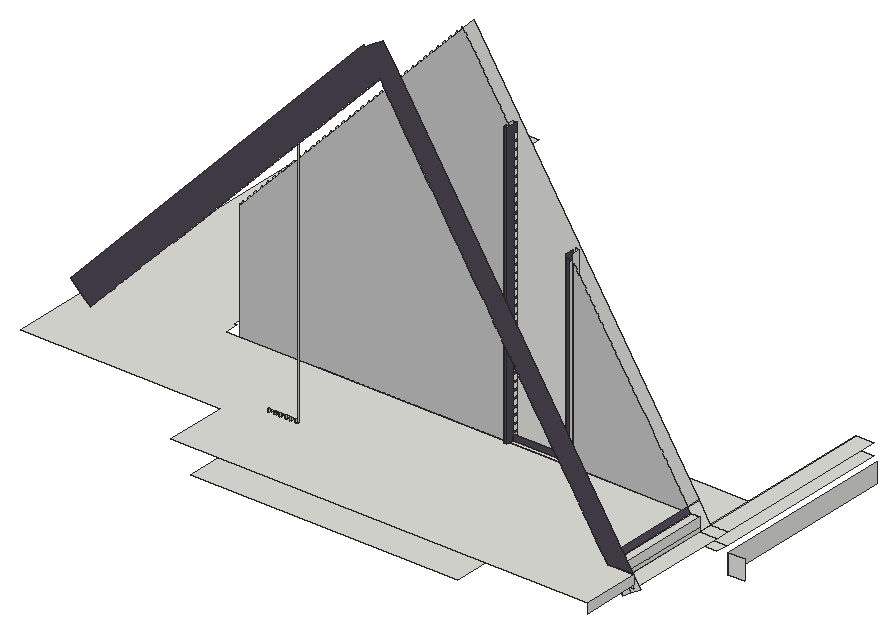
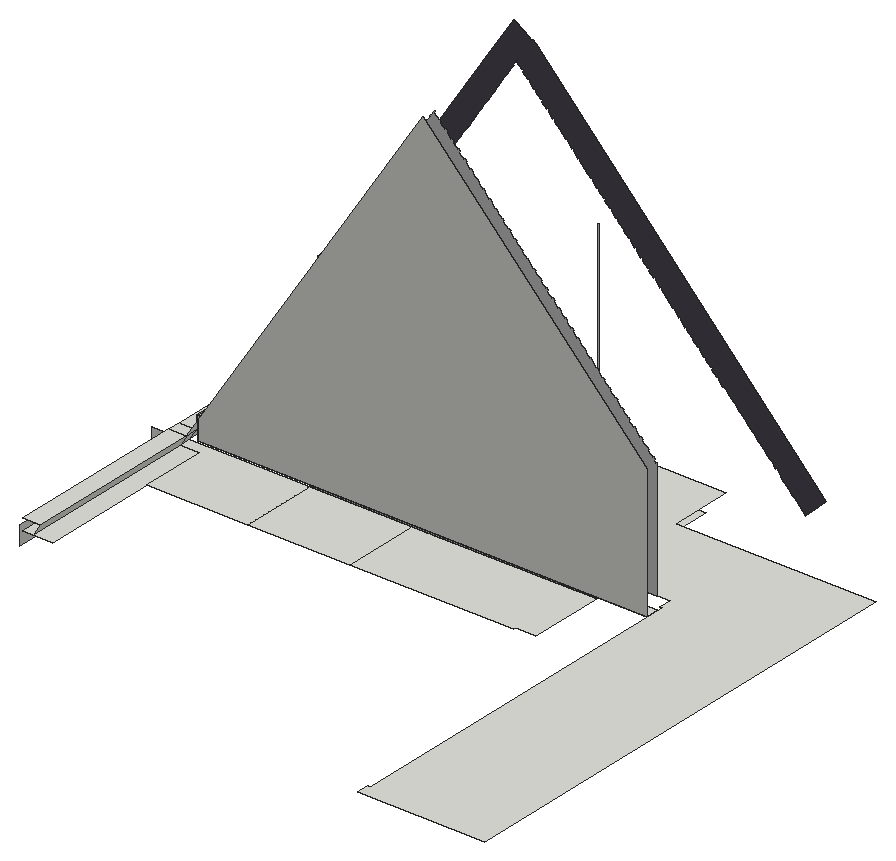
# SketchUp Ruby script. Lengths in inches.
U = 1.inch
M = Sketchup.active_model
def pt(a) = Geom::Point3d.new(a.map { |v| v * U })
def face(e, loops, mat)
  f = e.add_face(loops[0].map { |a| pt(a) })
  loops[1..].each { |l| e.add_face(l.map { |a| pt(a) }).erase! }
  f.material = f.back_material = mat if mat
  f
end
# faces: each face lists its corners as indices into pts; further lists are holes
def faces(e, pts, list, mat = nil) = list.each { |f| face(e, (f[0].is_a?(Array) ? f : [f]).map { |l| l.map { |i| pts[i] } }, mat) }
# xy, xz, yz: faces in a plane at the given z, y or x. An outline is a flat list of corners, or four numbers for a rectangle; further outlines are holes
def ring(l) = l.size == 4 ? [[l[0], l[1]], [l[2], l[1]], [l[2], l[3]], [l[0], l[3]]] : l.each_slice(2).to_a
def flat(e, list, mat, &to3) = list.each { |f| face(e, (f[0].is_a?(Array) ? f : [f]).map { |l| ring(l).map { |u, v| to3.(u, v) } }, mat) }
def xy(e, z, list, mat = nil) = flat(e, list, mat) { |x, y| [x, y, z] }
def xz(e, y, list, mat = nil) = flat(e, list, mat) { |x, z| [x, y, z] }
def yz(e, x, list, mat = nil) = flat(e, list, mat) { |y, z| [x, y, z] }
def lines(e, pts, list) = list.each { |a, b| e.add_line(pt(pts[a]), pt(pts[b])) }
# prism: a flat outline (further loops are holes) pulled along v
def prism(e, loops, v, mat = nil)
  f = face(e, loops, mat); d = Geom::Vector3d.new(v.map { |x| x * U })
  f.pushpull(f.normal.samedirection?(d) ? d.length : -d.length)
end
def box(e, o, s, mat = nil) = prism(e, [[o, [o[0] + s[0], o[1], o[2]], [o[0] + s[0], o[1] + s[1], o[2]], [o[0], o[1] + s[1], o[2]]]], [0, 0, s[2]], mat)
def at(x, y, z, deg = 0) = Geom::Transformation.translation(pt([x, y, z])) * Geom::Transformation.rotation(ORIGIN, Z_AXIS, deg.degrees)
def axes(o, x, y, z) = Geom::Transformation.new([*x, 0, *y, 0, *z, 0, *pt(o).to_a, 1])
def part(name) = M.definitions.add(name)
# library, detail: a bought-in or finely detailed component or shape, given as its bounding box
def library(name, o, s) = part(name).tap { |d| box(d.entities, o, s) }
def detail(e, o, s) = box(e.add_group.entities, o, s)
def put(e, d, t, mat = nil) = e.add_instance(d, t).tap { |i| i.material = mat if mat }
def group(e, t, mat = nil) = e.add_group.tap { |g| g.transformation = t; g.material = mat if mat }.entities
root = M.entities
M.materials.add("[Color M02]").color = [198, 198, 198]
M.materials.add("[Color M06]").color = [79, 71, 84]
c1 = library("A$C06767DEF\#1",[-8.3,1.21,0],[7.09,7.09,5.51])
xy(root,250.875,[[[1365.01,437.0625,1365.01,509.6875,1451.49,509.6875,1451.49,521.5625,1504.89,521.5625,1504.89,437.0625],[1470.93,456.39,1472.48,456.6,1473.93,457.2,1475.17,458.15,1476.12,459.39,1476.72,460.84,1476.93,462.39,1476.72,463.95,1476.12,465.39,1475.17,466.64,1473.93,467.59,1472.48,468.1875,1470.93,468.39,1469.375,468.1875,1467.93,467.59,1466.68,466.64,1465.73,465.39,1465.13,463.95,1464.93,462.39,1465.13,460.84,1465.73,459.39,1466.68,458.15,1467.93,457.2,1469.375,456.6],[1407.85,459.39,1409.4,459.6,1410.85,460.2,1412.09,461.15,1413.04,462.39,1413.64,463.84,1413.85,465.39,1413.64,466.95,1413.04,468.39,1412.09,469.64,1410.85,470.59,1409.4,471.1875,1407.85,471.39,1406.3,471.1875,1404.85,470.59,1403.61,469.64,1402.65,468.39,1402.05,466.95,1401.85,465.39,1402.05,463.84,1402.65,462.39,1403.61,461.15,1404.85,460.2,1406.3,459.6]]])
xy(root,251.0625,[[1365.01,509.6875,1451.49,521.5625],[1354.48,521.5625,1354.48,561.375,1365.24,561.375,1365.24,562.32,1451.49,562.32,1451.49,521.5625],[1451.49,521.5625,1504.89,562.32],[1504.89,521.5625,1504.89,562.32,1557.79,562.32,1557.79,527.76,1573.31,527.76,1573.31,521.5625],[1557.79,527.76,1573.31,623.84]])
xy(root,252.25,[[1470.93,456.39,1469.375,456.6,1467.93,457.2,1466.68,458.15,1465.73,459.39,1465.13,460.84,1464.93,462.39,1465.13,463.95,1465.73,465.39,1466.68,466.64,1467.93,467.59,1469.375,468.1875,1470.93,468.39,1472.48,468.1875,1473.93,467.59,1475.17,466.64,1476.12,465.39,1476.72,463.95,1476.93,462.39,1476.72,460.84,1476.12,459.39,1475.17,458.15,1473.93,457.2,1472.48,456.6]])
xy(root,252.375,[[1407.85,459.39,1406.3,459.6,1404.85,460.2,1403.61,461.15,1402.65,462.39,1402.05,463.84,1401.85,465.39,1402.05,466.95,1402.65,468.39,1403.61,469.64,1404.85,470.59,1406.3,471.1875,1407.85,471.39,1409.4,471.1875,1410.85,470.59,1412.09,469.64,1413.04,468.39,1413.64,466.95,1413.85,465.39,1413.64,463.84,1413.04,462.39,1412.09,461.15,1410.85,460.2,1409.4,459.6]])
xy(root,257.0625,[[1563.99,467.1875,1573.31,521.5625],[1322.96,521.5625,1557.92,528.48],[1563.99,521.5625,1573.31,528.48],[1563.99,528.48,1573.31,623.84]])
xy(root,259.68,[[1371.61,480.14,1373.93,480.77],[1374.53,480.14,1376.84,480.77],[1377.4375,480.14,1379.75,480.77],[1380.35,480.14,1382.66,480.77],[1383.26,480.14,1385.58,480.77]])
xy(root,262,[[1371.61,480.14,1373.93,480.77],[1374.53,480.14,1376.84,480.77],[1377.4375,480.14,1379.75,480.77],[1380.35,480.14,1382.66,480.77],[1383.26,480.14,1385.58,480.77]])
xy(root,262.73,[[1371.64,480.14,1373.96,480.77],[1374.56,480.14,1376.87,480.77],[1377.47,480.14,1379.78,480.77],[1380.38,480.14,1382.69,480.77],[1383.29,480.14,1385.6,480.77]])
xy(root,263.89,[[[1354.48,437.0625,1573.31,437.0625,1573.31,467.1875,1563.99,467.1875,1563.99,521.5625,1497.36,521.5625,1497.36,519.6875,1495.49,519.6875,1495.49,521.5625,1464.52,521.5625,1464.52,519.6875,1462.77,519.6875,1462.77,521.5625,1316.04,521.5625,1316.04,528.48,1314.46,528.48,1314.46,719.59,1316.04,719.59,1316.04,726.125,1249.48,726.125,1249.48,469.875,1354.48,469.875],[1317.4375,480.14,1386.75,480.77]],[1462.77,519.6875,1464.52,521.5625],[1495.49,519.6875,1497.36,521.5625],[1462.77,521.5625,1464.52,526.125],[1464.52,521.5625,1495.49,523.75],
  [1495.49,521.5625,1497.36,526.125]])
xy(root,265.04,[[1371.64,480.14,1373.96,480.77],[1374.56,480.14,1376.87,480.77],[1377.47,480.14,1379.78,480.77],[1380.38,480.14,1382.69,480.77],[1383.29,480.14,1385.6,480.77]])
xz(root,467.1875,[[1567.23,252.01,1571.28,254.61,1569.71,257.0625,1563.99,257.0625],[1571.28,254.61,1576.55,257.98,1573.31,263.03,1573.31,257.0625,1569.71,257.0625],[1563.99,257.0625,1569.71,258.95],[1569.71,257.0625,1573.31,258.95],[1563.99,258.95,1569.71,263.89],
  [1569.71,258.95,1573.31,258.95,1573.31,263.03,1572.76,263.89,1569.71,263.89],[1573.31,263.03,1572.76,263.89,1573.31,263.89]])
xz(root,467.1875,[[1563.99,257.0625,1563.99,263.89,1572.76,263.89,1449.33,456.41,1441.66,468.38,1436.39,465.01,1432,462.19,1431.44,462.72,1430.11,461.31,1277.91,299.61,1285.45,292.52,1288.59,289.56,1291.01,292.13,1291.88,293.0625,1294.3,295.64,1295.18,296.57,1297.6,299.14,1298.48,300.07,1300.9,302.64,1301.78,303.58,1301.55,303.79,1303.97,306.36,1304.2,306.15,1305.08,307.08,1304.85,307.29,1307.27,309.87,1307.5,309.65,1308.375,310.59,1310.8,313.16,1311.68,314.09,1314.1,316.66,1314.97,317.59,1317.39,320.17,1318.27,321.1,1320.69,323.67,1321.57,324.6,1323.99,327.17,1324.87,328.11,1327.29,330.68,1328.17,331.61,1330.59,334.18,1331.47,335.11,1331.92,334.6875,1334.34,337.26,1333.89,337.6875,1334.76,338.62,1335.22,338.19,1337.64,340.76,1337.1875,341.19,1338.0625,342.125,1338.52,341.69,1340.94,344.27,1340.48,344.7,1341.36,345.63,1341.82,345.2,1344.24,347.77,1343.78,348.2,1344.66,349.13,1345.12,348.7,1347.54,351.28,1347.08,351.7,1347.96,352.64,1348.41,352.21,1350.84,354.78,1350.38,355.21,1351.26,356.14,1351.71,355.71,1354.13,358.28,1353.68,358.71,1354.56,359.64,1355.01,359.22,1357.43,361.79,1356.98,362.22,1357.85,363.15,1358.31,362.72,1360.73,365.29,1360.28,365.72,1361.15,366.65,1361.61,366.22,1364.03,368.8,1363.57,369.23,1364.45,370.16,1364.91,369.73,1367.33,372.3,1366.87,372.73,1367.75,373.66,1368.21,373.23,1370.625,375.81,1370.17,376.23,1371.05,377.17,1371.5,376.74,1373.92,379.31,1373.47,379.74,1374.35,380.67,1374.8,380.24,1377.22,382.8125,1376.77,383.24,1377.65,384.17,1378.1,383.75,1380.52,386.32,1380.07,386.75,1380.94,387.68,1381.4,387.25,1383.82,389.82,1383.37,390.25,1384.24,391.18,1384.7,390.75,1387.12,393.33,1386.66,393.75,1387.54,394.6875,1388,394.26,1390.42,396.83,1389.96,397.26,1390.84,398.19,1391.3,397.76,1393.72,400.34,1393.26,400.76,1394.14,401.7,1394.59,401.27,1397.01,403.84,1396.56,404.27,1397.4375,405.2,1397.89,404.77,1400.3125,407.34,1399.86,407.77,1400.74,408.7,1401.19,408.28,1403.61,410.85,1403.16,411.28,1404.03,412.21,1404.49,411.78,1406.91,414.35,1406.46,414.78,1407.33,415.71,1407.79,415.28,1410.21,417.86,1409.75,418.28,1410.63,419.22,1411.09,418.79,1413.51,421.36,1413.05,421.79,1413.93,422.72,1414.38,422.29,1416.81,424.86,1416.35,425.29,1417.23,426.23,1417.68,425.8,1420.1,428.37,1419.65,428.8,1420.53,429.73,1420.98,429.3,1423.4,431.875,1422.95,432.3,1423.83,433.23,1424.28,432.81,1426.7,435.38,1426.25,435.81,1427.125,436.74,1427.58,436.31,1430,438.88,1429.55,439.31,1430.42,440.24,1430.88,439.8125,1433.3,442.39,1432.84,442.8125,1433.72,443.75,1434.18,443.32,1436.6,445.89,1436.14,446.32,1437.02,447.25,1437.47,446.82,1439.9,449.39,1439.44,449.82,1439.71,450.11,1440.02,450.4375,1441.59,447.99,1442.09,447.21,1441.72,446.98,1443.41,444.33,1443.78,444.57,1444.28,443.79,1443.91,443.56,1445.61,440.91,1445.97,441.15,1446.47,440.375,1446.1,440.14,1447.8,437.49,1448.17,437.73,1448.66,436.95,1448.3,436.72,1449.99,434.07,1450.36,434.31,1450.86,433.53,1450.49,433.3,1452.18,430.65,1452.55,430.89,1453.05,430.11,1452.68,429.88,1454.375,427.23,1454.74,427.47,1455.24,426.69,1454.875,426.46,1456.57,423.8125,1456.9375,424.05,1457.43,423.27,1457.07,423.04,1458.76,420.39,1459.13,420.63,1459.63,419.85,1459.26,419.62,1460.95,416.97,1461.32,417.21,1461.82,416.43,1461.45,416.2,1463.15,413.55,1463.51,413.79,1464.01,413.01,1463.64,412.78,1465.34,410.13,1465.71,410.37,1466.2,409.59,1465.84,409.36,1467.53,406.71,1467.9,406.95,1468.4,406.17,1468.03,405.9375,1469.72,403.29,1470.09,403.53,1470.59,402.75,1470.22,402.52,1471.92,399.875,1472.28,400.11,1472.78,399.33,1472.41,399.1,1474.11,396.45,1474.48,396.69,1474.98,395.91,1474.61,395.68,1476.3,393.03,1476.67,393.27,1477.17,392.49,1476.8,392.26,1478.49,389.61,1478.86,389.85,1479.36,389.07,1478.99,388.84,1480.6875,386.19,1481.05,386.43,1481.55,385.65,1481.18,385.42,1482.88,382.77,1483.25,383.01,1483.75,382.23,1483.38,382,1485.07,379.35,1485.44,379.59,1485.9375,378.8125,1485.57,378.58,1487.26,375.93,1487.63,376.17,1488.13,375.39,1487.76,375.16,1489.46,372.51,1489.83,372.75,1490.32,371.97,1489.96,371.74,1491.65,369.09,1492.02,369.33,1492.65,368.34,1492.28,368.11,1493.98,365.46,1494.35,365.7,1494.98,364.71,1496.67,362.07,1497.31,361.08,1496.9375,360.85,1498.63,358.2,1499,358.4375,1499.63,357.45,1499.27,357.22,1500.96,354.57,1501.33,354.81,1501.96,353.82,1501.59,353.58,1503.29,350.94,1503.66,351.18,1504.29,350.19,1503.92,349.95,1505.61,347.3125,1505.98,347.55,1506.62,346.56,1506.25,346.32,1507.94,343.68,1508.3125,343.92,1508.94,342.93,1508.58,342.69,1510.27,340.05,1510.64,340.29,1511.17,339.46,1510.8,339.22,1512.5,336.58,1512.86,336.8125,1513.4,335.98,1513.03,335.75,1514.72,333.11,1515.09,333.34,1515.62,332.51,1515.25,332.28,1516.95,329.63,1517.32,329.87,1517.85,329.04,1517.48,328.8,1519.18,326.16,1519.54,326.4,1520.08,325.57,1519.71,325.33,1521.4,322.6875,1521.77,322.92,1522.3,322.09,1521.93,321.86,1523.63,319.21,1524,319.45,1524.53,318.62,1524.16,318.38,1525.85,315.74,1526.22,315.98,1526.75,315.15,1526.39,314.91,1528.08,312.27,1528.45,312.51,1528.98,311.68,1528.61,311.44,1530.31,308.8,1530.68,309.03,1531.21,308.2,1530.84,307.97,1532.53,305.32,1532.9,305.56,1533.43,304.73,1533.07,304.49,1534.76,301.85,1535.13,302.09,1535.66,301.26,1535.4,301.09,1537.09,298.45,1537.35,298.61,1537.89,297.79,1537.62,297.62,1539.32,294.97,1539.58,295.14,1540.11,294.3125,1539.85,294.14,1541.54,291.5,1541.81,291.67,1542.34,290.84,1542.08,290.67,1543.77,288.03,1544.03,288.2,1544.56,287.37,1544.3,287.2,1546,284.56,1546.26,284.72,1546.79,283.89,1546.53,283.73,1548.22,281.08,1548.49,281.25,1549.02,280.42,1548.75,280.25,1550.45,277.61,1550.71,277.78,1551.24,276.95,1550.98,276.78,1552.68,274.14,1552.9375,274.31,1553.47,273.48,1553.21,273.31,1554.9,270.67,1555.16,270.83,1555.7,270,1555.43,269.84,1557.13,267.19,1557.39,267.36,1557.92,266.53,1557.66,266.36,1559.35,263.72,1559.62,263.89]],"[Color M06]")
xz(root,480.14,[[1386.17,258.95,1386.75,263.89],[1371.64,262.73,1373.96,263.89],[1374.56,262.73,1376.87,263.89],[1377.47,262.73,1379.78,263.89],[1380.38,262.73,1382.69,263.89],
  [1383.29,262.73,1385.6,263.89]])
xz(root,480.77,[[1371.64,262.73,1373.96,263.89],[1374.56,262.73,1376.87,263.89],[1377.47,262.73,1379.78,263.89],[1380.38,262.73,1382.69,263.89],[1383.29,262.73,1385.6,263.89]])
xz(root,509.6875,[[1365.01,250.875,1451.49,251.0625]])
xz(root,519.6875,[[1462.77,263.89,1464.52,412.22],[1495.49,263.89,1497.36,263.89,1497.36,360.99,1496.99,360.76,1496.9375,360.85,1497.31,361.08,1496.67,362.07,1496.3,361.83,1495.49,363.11]],"[Color M06]")
xz(root,521.5625,[[1451.49,250.875,1504.89,251.0625],[1365.01,251.0625,1504.89,257.0625],[1365.01,257.0625,1504.89,258.95],[1504.89,257.0625,1557.92,258.95],[1557.92,257.0625,1563.99,257.0625,1562.78,258.95,1557.92,258.95],
  [1563.99,257.0625,1562.78,258.95,1563.99,258.95],[1365.01,258.95,1504.89,263.89],[1504.89,258.95,1557.92,263.89],[1557.92,258.95,1562.78,258.95,1559.62,263.89,1559.35,263.72,1559.25,263.89,1557.92,263.89],[1562.78,258.95,1559.62,263.89,1562.78,263.89],
  [1562.78,258.95,1563.99,263.89],[1559.35,263.72,1559.25,263.89,1559.62,263.89],[1557.92,263.89,1559.25,263.89,1557.92,265.95],[1559.25,263.89,1559.62,263.89,1557.92,266.53,1557.92,265.95]])
xz(root,521.5625,[[1322.96,263.89,1462.77,263.89,1462.77,412.22,1464,412.22,1463.7,412.6875,1464.07,412.92,1463.51,413.79,1463.15,413.55,1461.96,415.41,1461.51,416.11,1461.875,416.34,1461.32,417.21,1460.95,416.97,1459.77,418.83,1459.32,419.53,1459.68,419.76,1459.13,420.63,1458.76,420.39,1457.57,422.25,1457.12,422.95,1457.49,423.18,1456.9375,424.05,1456.57,423.8125,1455.38,425.67,1454.93,426.37,1455.3,426.6,1454.74,427.47,1454.375,427.23,1453.1875,429.09,1452.74,429.79,1453.11,430.02,1452.55,430.89,1452.18,430.65,1451,432.51,1450.55,433.21,1450.91,433.44,1450.36,434.31,1449.99,434.07,1448.8,435.93,1448.35,436.63,1448.72,436.86,1448.17,437.73,1447.8,437.49,1446.61,439.35,1446.16,440.05,1446.53,440.28,1445.97,441.15,1445.61,440.91,1444.42,442.77,1443.97,443.47,1444.34,443.7,1443.78,444.57,1443.41,444.33,1442.22,446.1875,1441.77,446.89,1442.14,447.125,1441.59,447.99,1441.22,447.75,1440.03,449.61,1439.71,450.11,1439.44,449.82,1439.9,449.39,1437.47,446.82,1437.02,447.25,1436.14,446.32,1436.6,445.89,1434.18,443.32,1433.72,443.75,1432.84,442.8125,1433.3,442.39,1430.88,439.8125,1430.42,440.24,1429.55,439.31,1430,438.88,1427.58,436.31,1427.125,436.74,1426.25,435.81,1426.7,435.38,1424.28,432.81,1423.83,433.23,1422.95,432.3,1423.4,431.875,1420.98,429.3,1420.53,429.73,1419.65,428.8,1420.1,428.37,1417.68,425.8,1417.23,426.23,1416.35,425.29,1416.81,424.86,1414.38,422.29,1413.93,422.72,1413.05,421.79,1413.51,421.36,1411.09,418.79,1410.63,419.22,1409.75,418.28,1410.21,417.86,1407.79,415.28,1407.33,415.71,1406.46,414.78,1406.91,414.35,1404.49,411.78,1404.03,412.21,1403.16,411.28,1403.61,410.85,1401.19,408.28,1400.74,408.7,1399.86,407.77,1400.3125,407.34,1397.89,404.77,1397.4375,405.2,1396.56,404.27,1397.01,403.84,1394.59,401.27,1394.14,401.7,1393.26,400.76,1393.72,400.34,1391.3,397.76,1390.84,398.19,1389.96,397.26,1390.42,396.83,1388,394.26,1387.54,394.6875,1386.66,393.75,1387.12,393.33,1384.7,390.75,1384.24,391.18,1383.37,390.25,1383.82,389.82,1381.4,387.25,1380.94,387.68,1380.07,386.75,1380.52,386.32,1378.1,383.75,1377.65,384.17,1376.77,383.24,1377.22,382.8125,1374.8,380.24,1374.35,380.67,1373.47,379.74,1373.92,379.31,1371.5,376.74,1371.05,377.17,1370.17,376.23,1370.625,375.81,1368.21,373.23,1367.75,373.66,1366.87,372.73,1367.33,372.3,1364.91,369.73,1364.45,370.16,1363.57,369.23,1364.03,368.8,1361.61,366.22,1361.15,366.65,1360.28,365.72,1360.73,365.29,1358.31,362.72,1357.85,363.15,1356.98,362.22,1357.43,361.79,1355.01,359.22,1354.56,359.64,1353.68,358.71,1354.13,358.28,1351.71,355.71,1351.26,356.14,1350.38,355.21,1350.84,354.78,1348.41,352.21,1347.96,352.64,1347.08,351.7,1347.54,351.28,1345.12,348.7,1344.66,349.13,1343.78,348.2,1344.24,347.77,1341.82,345.2,1341.36,345.63,1340.48,344.7,1340.94,344.27,1338.52,341.69,1338.0625,342.125,1337.1875,341.19,1337.64,340.76,1337.04,340.125,1336.64,339.7,1335.22,338.19,1334.76,338.62,1333.89,337.6875,1334.34,337.26,1331.92,334.6875,1331.47,335.11,1330.59,334.18,1331.04,333.75,1328.62,331.18,1328.17,331.61,1327.29,330.68,1327.75,330.25,1325.32,327.68,1324.87,328.11,1323.99,327.17,1324.45,326.75,1323.42,325.65,1322.96,326.08],[1497.36,263.89,1557.92,263.89,1557.92,265.95,1557.66,266.36,1557.92,266.53,1557.39,267.36,1557.13,267.19,1555.43,269.84,1555.7,270,1555.16,270.83,1554.9,270.67,1553.21,273.31,1553.47,273.48,1552.9375,274.31,1552.68,274.14,1550.98,276.78,1551.24,276.95,1550.71,277.78,1550.45,277.61,1548.75,280.25,1549.02,280.42,1548.49,281.25,1548.22,281.08,1546.53,283.73,1546.79,283.89,1546.26,284.72,1546,284.56,1544.3,287.2,1544.56,287.37,1544.03,288.2,1543.77,288.03,1542.08,290.67,1542.34,290.84,1541.81,291.67,1541.54,291.5,1539.85,294.14,1540.11,294.3125,1539.58,295.14,1537.89,297.79,1537.35,298.61,1535.66,301.26,1535.13,302.09,1534.76,301.85,1533.07,304.49,1533.43,304.73,1532.9,305.56,1532.53,305.32,1530.84,307.97,1531.21,308.2,1530.68,309.03,1530.31,308.8,1528.61,311.44,1528.98,311.68,1528.45,312.51,1528.08,312.27,1526.39,314.91,1526.75,315.15,1526.22,315.98,1525.85,315.74,1524.16,318.38,1524.53,318.62,1524,319.45,1523.63,319.21,1521.93,321.86,1522.3,322.09,1521.77,322.92,1521.4,322.6875,1519.71,325.33,1520.08,325.57,1519.54,326.4,1519.18,326.16,1517.48,328.8,1517.85,329.04,1517.32,329.87,1516.95,329.63,1515.25,332.28,1515.62,332.51,1515.09,333.34,1514.72,333.11,1513.03,335.75,1513.4,335.98,1512.86,336.8125,1512.5,336.58,1510.8,339.22,1511.17,339.46,1510.74,340.125,1510.64,340.29,1510.27,340.05,1508.58,342.69,1508.94,342.93,1508.3125,343.92,1507.94,343.68,1506.25,346.32,1506.62,346.56,1505.98,347.55,1505.61,347.3125,1503.92,349.95,1504.29,350.19,1503.66,351.18,1503.29,350.94,1501.59,353.58,1501.96,353.82,1501.33,354.81,1500.96,354.57,1499.27,357.22,1499.63,357.45,1499,358.4375,1498.63,358.2,1497.36,360.18]],"[Color M02]")
xz(root,523.31,[[1577.59,240.88,1586.28,251.0625]])
xz(root,523.75,[[1464.52,263.89,1495.49,267.02]],"[Color M06]")
xz(root,526.125,[[1462.77,263.89,1464.52,412.22],[1495.49,263.89,1497.36,363.92]])
xz(root,528.48,[[1322.96,257.0625,1322.96,326.08,1440.02,450.4375,1557.92,266.53,1557.92,257.0625]])
yz(root,1371.04,[[480.14,262.73,480.77,265.04]])
yz(root,1371.61,[[480.14,259.68,480.77,262]])
yz(root,1371.64,[[480.14,262.73,480.77,265.04]])
yz(root,1373.93,[[480.14,259.68,480.77,262]])
yz(root,1373.96,[[480.14,262.73,480.77,265.04]])
yz(root,1374.53,[[480.14,259.68,480.77,262]])
yz(root,1374.56,[[480.14,262.73,480.77,265.04]])
yz(root,1376.84,[[480.14,259.68,480.77,262]])
yz(root,1376.87,[[480.14,262.73,480.77,265.04]])
yz(root,1377.4375,[[480.14,259.68,480.77,262]])
yz(root,1377.47,[[480.14,262.73,480.77,265.04]])
yz(root,1379.75,[[480.14,259.68,480.77,262]])
yz(root,1379.78,[[480.14,262.73,480.77,265.04]])
yz(root,1380.35,[[480.14,259.68,480.77,262]])
yz(root,1380.38,[[480.14,262.73,480.77,265.04]])
yz(root,1382.66,[[480.14,259.68,480.77,262]])
yz(root,1382.69,[[480.14,262.73,480.77,265.04]])
yz(root,1383.26,[[480.14,259.68,480.77,262]])
yz(root,1383.29,[[480.14,262.73,480.77,265.04]])
yz(root,1385.58,[[480.14,259.68,480.77,262]])
yz(root,1385.6,[[480.14,262.73,480.77,265.04]])
yz(root,1386.75,[[480.14,258.95,480.77,263.89],[480.14,263.89,480.77,397.75]])
yz(root,1451.49,[[509.6875,250.875,521.5625,251.0625]])
yz(root,1462.77,[[521.5625,263.89,526.125,412.22]])
yz(root,1462.77,[[519.6875,263.89,521.5625,412.22]],"[Color M06]")
yz(root,1464.52,[[523.75,263.89,526.125,267.02]])
yz(root,1464.52,[[519.6875,263.89,523.75,263.89,523.75,267.02,526.125,267.02,526.125,267.83,523.75,267.83,523.75,270.95,526.125,270.95,526.125,271.76,523.75,271.76,523.75,274.89,526.125,274.89,526.125,275.7,523.75,275.7,523.75,278.83,526.125,278.83,526.125,279.64,523.75,279.64,523.75,282.77,526.125,282.77,526.125,283.58,523.75,283.58,523.75,286.7,526.125,286.7,526.125,287.51,523.75,287.51,523.75,290.64,526.125,290.64,526.125,291.45,523.75,291.45,523.75,294.58,526.125,294.58,526.125,295.39,523.75,295.39,523.75,298.52,526.125,298.52,526.125,299.33,523.75,299.33,523.75,302.45,526.125,302.45,526.125,303.26,523.75,303.26,523.75,306.39,526.125,306.39,526.125,307.2,523.75,307.2,523.75,310.33,526.125,310.33,526.125,311.14,523.75,311.14,523.75,314.27,526.125,314.27,526.125,315.08,524.25,315.08,524.25,318.2,526.125,318.2,526.125,319.01,524.25,319.01,524.25,322.14,526.125,322.14,526.125,322.89,524.25,322.89,524.25,326.02,526.125,326.02,526.125,326.76,524.25,326.76,524.25,329.89,526.125,329.89,526.125,330.64,524.25,330.64,524.25,333.77,526.125,333.77,526.125,334.51,524.25,334.51,524.25,337.64,526.125,337.64,526.125,338.39,524.25,338.39,524.25,341.52,526.125,341.52,526.125,341.93,524.25,341.93,524.25,345.06,526.125,345.06,526.125,346,524.25,346,524.25,349.12,526.125,349.12,526.125,350.06,524.25,350.06,524.25,353.18,526.125,353.18,526.125,354.12,524.25,354.12,524.25,357.25,526.125,357.25,526.125,358.06,524.25,358.06,524.25,361.18,526.125,361.18,526.125,362,524.25,362,524.25,365.12,526.125,365.12,526.125,366.25,524.25,366.25,524.25,369.37,526.125,369.37,526.125,370.5,524.25,370.5,524.25,373.62,526.125,373.62,526.125,374.75,524.25,374.75,524.25,377.87,526.125,377.87,526.125,379,524.25,379,524.25,382.12,526.125,382.12,526.125,383.25,524.25,383.25,524.25,386.37,526.125,386.37,526.125,387.5,524.25,387.5,524.25,390.62,526.125,390.62,526.125,391.75,524.25,391.75,524.25,394.87,526.125,394.87,526.125,396,524.25,396,524.25,399.12,526.125,399.12,526.125,400.25,524.25,400.25,524.25,403.37,526.125,403.37,526.125,404.5,524.25,404.5,524.25,407.62,526.125,407.62,526.125,412.22,519.6875,412.22]],"[Color M06]")
yz(root,1495.49,[[523.75,263.89,526.125,267.02]])
yz(root,1495.49,[[519.6875,263.89,519.6875,363.92,524.25,363.92,524.25,362,526.125,362,526.125,361.18,524.25,361.18,524.25,358.06,526.125,358.06,526.125,357.25,524.25,357.25,524.25,354.12,526.125,354.12,526.125,353.18,524.25,353.18,524.25,350.06,526.125,350.06,526.125,349.12,524.25,349.12,524.25,346,526.125,346,526.125,345.06,524.25,345.06,524.25,341.93,526.125,341.93,526.125,341.52,524.25,341.52,524.25,338.39,526.125,338.39,526.125,337.64,524.25,337.64,524.25,334.51,526.125,334.51,526.125,333.77,524.25,333.77,524.25,330.64,526.125,330.64,526.125,329.89,524.25,329.89,524.25,326.76,526.125,326.76,526.125,326.02,524.25,326.02,524.25,322.89,526.125,322.89,526.125,322.14,524.25,322.14,524.25,319.01,526.125,319.01,526.125,318.2,524.25,318.2,524.25,315.08,526.125,315.08,526.125,314.27,523.75,314.27,523.75,311.14,526.125,311.14,526.125,310.33,523.75,310.33,523.75,307.2,526.125,307.2,526.125,306.39,523.75,306.39,523.75,303.26,526.125,303.26,526.125,302.45,523.75,302.45,523.75,299.33,526.125,299.33,526.125,298.52,523.75,298.52,523.75,295.39,526.125,295.39,526.125,294.58,523.75,294.58,523.75,291.45,526.125,291.45,526.125,290.64,523.75,290.64,523.75,287.51,526.125,287.51,526.125,286.7,523.75,286.7,523.75,283.58,526.125,283.58,526.125,282.77,523.75,282.77,523.75,279.64,526.125,279.64,526.125,278.83,523.75,278.83,523.75,275.7,526.125,275.7,526.125,274.89,523.75,274.89,523.75,271.76,526.125,271.76,526.125,270.95,523.75,270.95,523.75,267.83,526.125,267.83,526.125,267.02,523.75,267.02,523.75,263.89]],"[Color M06]")
yz(root,1497.36,[[519.6875,263.89,521.5625,360.99],[521.5625,263.89,526.125,363.92]])
yz(root,1557.92,[[521.5625,257.0625,528.48,266.53]])
yz(root,1563.99,[[467.1875,257.0625,521.5625,258.95],[467.1875,258.95,521.5625,263.89]])
yz(root,1573.31,[[437.0625,258.95,467.1875,263.89]])
yz(root,1577.59,[[523.31,240.88,620.37,251.0625]])
p = [[1470.93,456.39,250.875],[1469.375,456.6,250.875],[1469.375,456.6,252.25],[1470.93,456.39,252.25],[1472.48,456.6,250.875],[1472.48,456.6,252.25],
  [1467.93,457.2,250.875],[1467.93,457.2,252.25],[1473.93,457.2,250.875],[1473.93,457.2,252.25],[1466.68,458.15,250.875],[1466.68,458.15,252.25],
  [1475.17,458.15,250.875],[1475.17,458.15,252.25],[1465.73,459.39,250.875],[1465.73,459.39,252.25],[1476.12,459.39,250.875],[1476.12,459.39,252.25],
  [1407.85,459.39,250.875],[1406.3,459.6,250.875],[1406.3,459.6,252.375],[1407.85,459.39,252.375],[1409.4,459.6,250.875],[1409.4,459.6,252.375],
  [1465.13,460.84,250.875],[1465.13,460.84,252.25],[1476.72,460.84,250.875],[1476.72,460.84,252.25],[1404.85,460.2,250.875],[1404.85,460.2,252.375],
  [1410.85,460.2,250.875],[1410.85,460.2,252.375],[1403.61,461.15,250.875],[1403.61,461.15,252.375],[1412.09,461.15,250.875],[1412.09,461.15,252.375],
  [1464.93,462.39,250.875],[1464.93,462.39,252.25],[1476.93,462.39,250.875],[1476.93,462.39,252.25],[1402.65,462.39,250.875],[1402.65,462.39,252.375],
  [1413.04,462.39,250.875],[1413.04,462.39,252.375],[1402.05,463.84,250.875],[1402.05,463.84,252.375],[1413.64,463.84,250.875],[1413.64,463.84,252.375],
  [1465.13,463.95,250.875],[1465.13,463.95,252.25],[1476.72,463.95,250.875],[1476.72,463.95,252.25],[1401.85,465.39,250.875],[1401.85,465.39,252.375],
  [1413.85,465.39,250.875],[1413.85,465.39,252.375],[1465.73,465.39,250.875],[1465.73,465.39,252.25],[1476.12,465.39,250.875],[1476.12,465.39,252.25],
  [1402.05,466.95,250.875],[1402.05,466.95,252.375],[1413.64,466.95,250.875],[1413.64,466.95,252.375],[1466.68,466.64,250.875],[1466.68,466.64,252.25],
  [1475.17,466.64,250.875],[1475.17,466.64,252.25],[1467.93,467.59,250.875],[1467.93,467.59,252.25],[1473.93,467.59,250.875],[1473.93,467.59,252.25],
  [1402.65,468.39,250.875],[1402.65,468.39,252.375],[1413.04,468.39,250.875],[1413.04,468.39,252.375],[1469.375,468.1875,250.875],[1469.375,468.1875,252.25],
  [1472.48,468.1875,250.875],[1472.48,468.1875,252.25],[1470.93,468.39,250.875],[1470.93,468.39,252.25],[1403.61,469.64,250.875],[1403.61,469.64,252.375],
  [1412.09,469.64,250.875],[1412.09,469.64,252.375],[1404.85,470.59,250.875],[1404.85,470.59,252.375],[1410.85,470.59,250.875],[1410.85,470.59,252.375],
  [1406.3,471.1875,250.875],[1406.3,471.1875,252.375],[1409.4,471.1875,250.875],[1409.4,471.1875,252.375],[1407.85,471.39,250.875],[1407.85,471.39,252.375],
  [1563.99,467.1875,257.0625],[1563.99,521.5625,257.0625],[1567.23,521.5625,252.01],[1567.23,467.1875,252.01],[1563.99,528.48,257.0625],[1567.23,528.48,252.01],
  [1563.99,623.84,257.0625],[1567.23,623.84,252.01],[1559.62,467.1875,263.89],[1559.62,521.5625,263.89],[1562.78,521.5625,258.95],[1557.92,528.48,266.53],
  [1557.92,521.5625,266.53],[1557.66,521.5625,266.36],[1557.92,521.5625,265.95],[1559.25,521.5625,263.89],[1559.35,521.5625,263.72],[1559.35,467.1875,263.72],
  [1557.66,467.1875,266.36]]
faces(root,p,[[0,1,2,3],[4,0,3,5],[1,6,7,2],[8,4,5,9],[6,10,11,7],[12,8,9,13],[10,14,15,11],[16,12,13,17],
  [18,19,20,21],[22,18,21,23],[14,24,25,15],[26,16,17,27],[19,28,29,20],[30,22,23,31],[28,32,33,29],[34,30,31,35],
  [24,36,37,25],[38,26,27,39],[32,40,41,33],[42,34,35,43],[40,44,45,41],[46,42,43,47],[36,48,49,37],[50,38,39,51],
  [44,52,53,45],[54,46,47,55],[48,56,57,49],[58,50,51,59],[52,60,61,53],[62,54,55,63],[56,64,65,57],[66,58,59,67],
  [64,68,69,65],[70,66,67,71],[60,72,73,61],[74,62,63,75],[68,76,77,69],[78,70,71,79],[76,80,81,77],[80,78,79,81],
  [72,82,83,73],[84,74,75,85],[82,86,87,83],[88,84,85,89],[86,90,91,87],[92,88,89,93],[90,94,95,91],[94,92,93,95],
  [96,97,98,99],[97,100,101,98],[100,102,103,101],[96,104,105,106,97],[100,107,108,105,106,97],[105,104,113,112]])
faces(root,p,[[109,110,111,112,113,114]],"[Color M06]")
put(root,c1,axes([1413.45,464.17,249.52],[1.14885,0,0],[0,0.84644,0],[0,0,0.5175]))
put(root,c1,axes([1477.51,458.37,248.02],[1.14885,0,0],[0,0.84644,0],[0,0,0.5175]))
